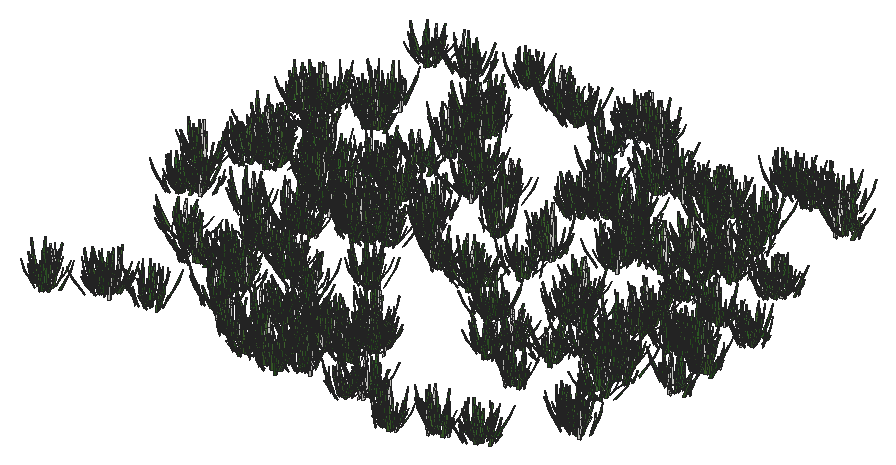
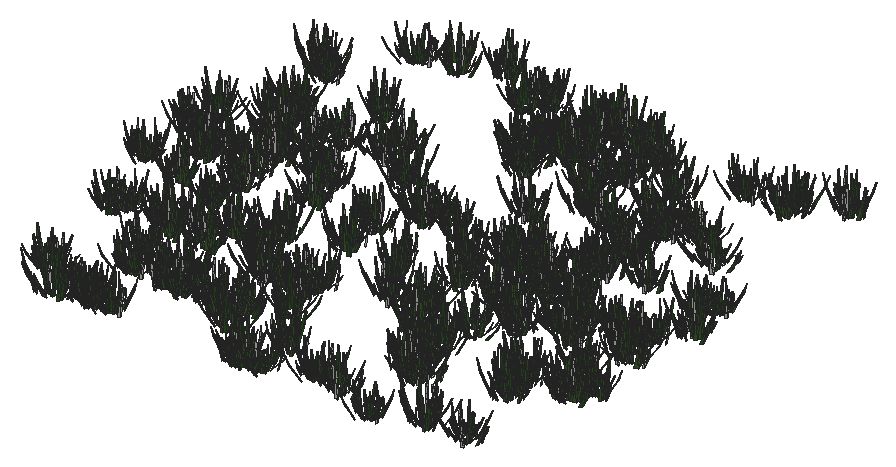
# SketchUp Ruby script. Lengths in inches.
U = 1.inch
M = Sketchup.active_model
def pt(a) = Geom::Point3d.new(a.map { |v| v * U })
def face(e, loops, mat)
  f = e.add_face(loops[0].map { |a| pt(a) })
  loops[1..].each { |l| e.add_face(l.map { |a| pt(a) }).erase! }
  f.material = f.back_material = mat if mat
  f
end
# faces: each face lists its corners as indices into pts; further lists are holes
def faces(e, pts, list, mat = nil) = list.each { |f| face(e, (f[0].is_a?(Array) ? f : [f]).map { |l| l.map { |i| pts[i] } }, mat) }
# xy, xz, yz: faces in a plane at the given z, y or x. An outline is a flat list of corners, or four numbers for a rectangle; further outlines are holes
def ring(l) = l.size == 4 ? [[l[0], l[1]], [l[2], l[1]], [l[2], l[3]], [l[0], l[3]]] : l.each_slice(2).to_a
def flat(e, list, mat, &to3) = list.each { |f| face(e, (f[0].is_a?(Array) ? f : [f]).map { |l| ring(l).map { |u, v| to3.(u, v) } }, mat) }
def xy(e, z, list, mat = nil) = flat(e, list, mat) { |x, y| [x, y, z] }
def xz(e, y, list, mat = nil) = flat(e, list, mat) { |x, z| [x, y, z] }
def yz(e, x, list, mat = nil) = flat(e, list, mat) { |y, z| [x, y, z] }
def lines(e, pts, list) = list.each { |a, b| e.add_line(pt(pts[a]), pt(pts[b])) }
# prism: a flat outline (further loops are holes) pulled along v
def prism(e, loops, v, mat = nil)
  f = face(e, loops, mat); d = Geom::Vector3d.new(v.map { |x| x * U })
  f.pushpull(f.normal.samedirection?(d) ? d.length : -d.length)
end
def box(e, o, s, mat = nil) = prism(e, [[o, [o[0] + s[0], o[1], o[2]], [o[0] + s[0], o[1] + s[1], o[2]], [o[0], o[1] + s[1], o[2]]]], [0, 0, s[2]], mat)
def at(x, y, z, deg = 0) = Geom::Transformation.translation(pt([x, y, z])) * Geom::Transformation.rotation(ORIGIN, Z_AXIS, deg.degrees)
def axes(o, x, y, z) = Geom::Transformation.new([*x, 0, *y, 0, *z, 0, *pt(o).to_a, 1])
def part(name) = M.definitions.add(name)
# library, detail: a bought-in or finely detailed component or shape, given as its bounding box
def library(name, o, s) = part(name).tap { |d| box(d.entities, o, s) }
def detail(e, o, s) = box(e.add_group.entities, o, s)
def put(e, d, t, mat = nil) = e.add_instance(d, t).tap { |i| i.material = mat if mat }
def group(e, t, mat = nil) = e.add_group.tap { |g| g.transformation = t; g.material = mat if mat }.entities
root = M.entities
M.materials.add("Material1").color = [58, 110, 58]
M.materials.add("Material10").color = [48, 100, 38]
M.materials.add("Material3").color = [68, 110, 58]
M.materials.add("Material4").color = [48, 90, 38]
M.materials.add("Material5").color = [68, 110, 48]
M.materials.add("Material6").color = [48, 90, 48]
M.materials.add("Material8").color = [58, 90, 38]
M.materials.add("Material9").color = [68, 100, 58]
c1 = part("grass00")
p = [[-0.6875,0.15,0],[-0.56,0.08,5.52],[-0.04,0.03,2.76],[0.48,-0.02,0],[0.35,-0.02,5.52],[-0.1,-0.14,5.52],
  [-0.12,0.65,8.37],[-0.42,0.65,8.37]]
faces(c1.entities,p,[[0,1,2,3],[3,2,4],[1,5,2],[5,4,2],[1,6,5],[4,5,6],[7,6,1]])
c2 = part("Group16\#1")
put(c2.entities,c1,axes([1.44,-0.61,-0.01],[0.05352,0.12609,0],[-0.10704,0.04543,0.07239],[0.06664,-0.02828,0.11628]),"Material6")
put(c2.entities,c1,axes([0.76,-0.15,-0.01],[0.04676,0.24062,0],[-0.23162,0.04501,0.06642],[0.0652,-0.01267,0.23595]),"Material3")
put(c2.entities,c1,axes([0.79,0.01,-0.01],[-0.00606,0.34651,0],[-0.34381,-0.00602,0.0432],[0.04319,0.00076,0.34386]))
put(c2.entities,c1,axes([1,0.23,-0.01],[-0.07192,0.31144,0],[-0.28722,-0.06632,0.1236],[0.12043,0.02781,0.29478]),"Material5")
put(c2.entities,c1,axes([1.66,0.77,-0.01],[-0.13828,0.29651,0],[-0.21551,-0.1005,0.22471],[0.20365,0.09498,0.23779]),"Material10")
put(c2.entities,c1,axes([0.6875,0.52,-0.01],[-0.18126,0.24051,0],[-0.22746,-0.17142,0.09788],[0.07817,0.05891,0.28481]),"Material5")
put(c2.entities,c1,axes([0.68,0.78,-0.01],[-0.215,0.18688,0],[-0.12385,-0.14248,0.21334],[0.13995,0.16101,0.18878]),"Material3")
put(c2.entities,c1,axes([0.56,1,-0.01],[-0.13756,0.07624,0],[-0.06159,-0.11112,0.0927],[0.04494,0.08108,0.12705]),"Material5")
put(c2.entities,c1,axes([0.2,0.64,-0.01],[-0.23729,0.07254,0],[-0.05711,-0.18681,0.153],[0.04473,0.14632,0.19535]),"Material10")
put(c2.entities,c1,axes([0.0625,0.72,-0.01],[-0.28874,0.02525,0],[-0.02179,-0.24916,0.14647],[0.01276,0.14591,0.25012]),"Material3")
put(c2.entities,c1,axes([-0.08,0.62,-0.01],[-0.34089,-0.04187,0],[0.03255,-0.26504,0.216],[-0.02633,0.21439,0.26703]),"Material10")
put(c2.entities,c1,axes([-0.34,0.98,-0.01],[-0.14314,-0.0493,0],[0.04397,-0.12769,0.06843],[-0.02228,0.0647,0.13505]),"Material10")
put(c2.entities,c1,axes([-0.87,1.45,-0.01],[-0.23488,-0.14114,0],[0.13761,-0.22901,0.06087],[-0.03135,0.05217,0.26717]))
put(c2.entities,c1,axes([-0.72,0.77,-0.01],[-0.14208,-0.13251,0],[0.07209,-0.0773,0.16301],[-0.11118,0.11922,0.1057]),"Material10")
put(c2.entities,c1,axes([-0.62,0.43,-0.01],[-0.14845,-0.21203,0],[0.18654,-0.13061,0.12304],[-0.10079,0.07057,0.22772]),"Material3")
put(c2.entities,c1,axes([-0.68,0.29,-0.01],[-0.13639,-0.32136,0],[0.31723,-0.13464,0.05579],[-0.05136,0.0218,0.34462]),"Material4")
put(c2.entities,c1,axes([-0.64,0.125,-0.01],[-0.0458,-0.23569,0],[0.22124,-0.043,0.08276],[-0.08124,0.01579,0.22538]),"Material1")
put(c2.entities,c1,axes([-1.6,-0.03,-0.01],[0.00576,-0.32897,0],[0.27526,0.00482,0.18018],[-0.18015,-0.00315,0.2753]),"Material5")
put(c2.entities,c1,axes([-1.36,-0.31,-0.01],[0.05718,-0.24765,0],[0.18172,0.04196,0.17267],[-0.16825,-0.03885,0.1865]),"Material10")
put(c2.entities,c1,axes([-1.54,-0.72,-0.01],[0.06537,-0.14017,0],[0.13555,0.06321,0.03939],[-0.0357,-0.01665,0.14956]))
put(c2.entities,c1,axes([-1.19,-0.9,-0.01],[0.09597,-0.12735,0],[0.11214,0.08451,0.07557],[-0.06035,-0.04548,0.14042]),"Material9")
put(c2.entities,c1,axes([-0.47,-0.54,-0.01],[0.11588,-0.10072,0],[0.0618,0.0711,0.12124],[-0.07953,-0.0915,0.0942]))
put(c2.entities,c1,axes([-0.47,-0.84,-0.01],[0.11927,-0.0661,0],[0.06603,0.11913,0.00646],[-0.00313,-0.00565,0.13621]),"Material5")
put(c2.entities,c1,axes([-0.38,-1.24,-0.01],[0.28037,-0.08571,0],[0.0618,0.20215,0.20315],[-0.05939,-0.19428,0.21139]),"Material9")
put(c2.entities,c1,axes([-0.06,-0.66,-0.01],[0.22719,-0.01987,0],[0.01247,0.14255,0.17758],[-0.01547,-0.17691,0.1431]),"Material8")
put(c2.entities,c1,axes([0.11,-0.89,-0.01],[0.14882,0.01828,0],[-0.01058,0.08611,0.12229],[0.01491,-0.12138,0.08676]),"Material6")
put(c2.entities,c1,axes([0.25,-0.72,-0.01],[0.20481,0.07053,0],[-0.06206,0.18022,0.10291],[0.03351,-0.0973,0.1906]),"Material6")
put(c2.entities,c1,axes([0.85,-1.42,-0.01],[0.16481,0.09904,0],[-0.09472,0.15762,0.05616],[0.02893,-0.04814,0.18389]),"Material5")
put(c2.entities,c1,axes([1.01,-1.09,-0.01],[0.21858,0.20385,0],[-0.17495,0.1876,0.15339],[0.10462,-0.11218,0.25652]),"Material10")
put(c2.entities,c1,axes([1.01,-0.71,-0.01],[0.08733,0.12473,0],[-0.06445,0.04512,0.13037],[0.1068,-0.07477,0.07867]),"Material6")
c3 = part("Group15\#1")
put(c3.entities,c2,at(0,0,0))
c4 = part("3darcstudiotree_grass00\#1")
put(c4.entities,c3,at(0,0,0))
put(root,c4,axes([282.91,152.13,0.25],[0.50441,0.65823,0],[-1.00099,0.52844,-0.00074],[-0.00102,0.00054,1.93092]))
put(root,c4,axes([289.35,143.61,0.25],[-0.72293,0.89093,0],[-0.97329,-0.54407,-0.0002],[-0.00027,-0.00015,1.96126]))
put(root,c4,axes([270.9375,158.43,0.25],[0.98465,-0.12149,0],[0.17275,0.96453,-0.00967],[0.00171,0.00957,1.41667]))
put(root,c4,axes([310.59,141.94,0.25],[-0.66862,-0.69978,0],[0.89555,-0.58948,-0.01126],[0.01023,-0.00673,1.32461]))
put(root,c4,axes([321.16,143.97,0.25],[-0.64412,0.82006,0],[-0.86954,-0.47051,-0.00573],[-0.00758,-0.0041,1.63969]))
put(root,c4,axes([331.48,126.1875,0.25],[1.05486,0.41518,0],[-0.38969,0.68208,-0.0026],[-0.00222,0.00389,1.81639]))
put(root,c4,axes([308.12,144.92,0.25],[1.05826,0.20589,0],[-0.22246,0.78769,-0.007],[-0.00256,0.00908,1.56436]))
put(root,c4,axes([275.06,101.88,0.25],[0.19274,0.85396,0],[-1.19074,0.18514,-0.00799],[-0.00978,0.00152,1.50733]))
put(root,c4,axes([269.4,123.27,0.25],[-1.12748,0.03644,0],[-0.03558,-0.7583,-0.00954],[-0.00057,-0.01224,1.41434]))
put(root,c4,axes([280.94,137.52,0.25],[-0.12026,-0.90289,0],[0.9301,-0.08535,-0.00454],[0.00819,-0.00075,1.6986]))
put(root,c4,axes([307.15,99.47,0.25],[-0.42808,-0.69918,0],[0.99835,-0.42109,-0.00876],[0.01015,-0.00428,1.45672]))
put(root,c4,axes([291.02,126.91,0.25],[0.95151,-0.32357,0],[0.35722,0.72367,-0.00746],[0.00458,0.00929,1.52751]))
put(root,c4,axes([293.13,130.49,0.25],[-0.53335,-0.60654,0],[0.85943,-0.52062,-0.00015],[0.00022,-0.00014,1.94435]))
put(root,c4,axes([270.78,140.02,0.25],[-1.00771,-0.1754,0],[0.24056,-0.95209,-0.00999],[0.00242,-0.00957,1.38276]))
put(root,c4,axes([287.26,115.55,0.25],[0.92934,-0.33875,0],[0.46115,0.87155,-0.00525],[0.00304,0.00574,1.64886]))
put(root,c4,axes([273.91,114.75,0.25],[1.28779,-0.10782,0],[0.12101,0.99564,-0.01121],[0.00122,0.01004,1.30781]))
put(root,c4,axes([312.21,152.58,0.25],[0.38901,0.72653,0],[-1.07347,0.39596,-0.00487],[-0.00632,0.00233,1.66894]))
put(root,c4,axes([290.12,102.31,0.25],[-0.67966,0.71325,0],[-0.73342,-0.48146,-0.01059],[-0.0119,-0.00781,1.33934]))
put(root,c4,axes([298.05,99.55,0.25],[0.27356,-0.98457,0],[1.03655,0.1984,-0.00305],[0.00494,0.00095,1.76865]))
put(root,c4,axes([284.49,147.29,0.25],[-0.09469,-0.83837,0],[1.12214,-0.08731,-0.00863],[0.01106,-0.00086,1.44957]))
put(root,c4,axes([281.7,160.85,0.25],[0.75518,0.45958,0],[-0.62327,0.70554,-0.01003],[-0.0077,0.00872,1.36834]))
put(root,c4,axes([328.78,143.63,0.25],[-0.91105,0.16514,0],[-0.20716,-0.78732,-0.01018],[-0.00304,-0.01156,1.35975]))
put(root,c4,axes([325.4,119.33,0.25],[1.09165,0.06839,0],[-0.09508,1.04561,-0.00004],[0,0.00005,1.93334]))
put(root,c4,axes([298.02,135.62,0.25],[-0.36557,1.02345,0],[-0.8678,-0.21354,-0.00114],[-0.00227,-0.00056,1.86907]))
put(root,c4,axes([305.18,134.9,0.25],[-0.30893,0.95853,0],[-1.11215,-0.24693,-0.00132],[-0.00206,-0.00046,1.858]))
put(root,c4,axes([292.13,107.28,0.25],[0.76845,0.56751,0],[-0.64535,0.60199,-0.00943],[-0.00899,0.00839,1.39243]))
put(root,c4,axes([271.72,132.0625,0.25],[1.0465,-0.407,0],[0.49619,0.87892,-0.00986],[0.00489,0.00867,1.36783]))
put(root,c4,axes([283.01,118.25,0.25],[-0.20632,-0.8847,0],[0.88885,-0.1428,-0.00678],[0.01135,-0.00182,1.54322]))
put(root,c4,axes([325.72,157.09,0.25],[-1.09338,0.54066,0],[-0.57925,-0.80699,-0.00882],[-0.00569,-0.00792,1.42641]))
put(root,c4,axes([299.33,106.58,0.25],[0.13337,-0.79747,0],[0.99583,0.11473,-0.0013],[0.00238,0.00027,1.85519]))
put(root,c4,axes([294.85,118.7,0.25],[0.94591,-0.15419,0],[0.20231,0.855,-0.00241],[0.00079,0.00334,1.79003]))
put(root,c4,axes([309.11,101.2,0.25],[-0.922,0.2214,0],[-0.33581,-0.96337,-0.00573],[-0.00211,-0.00605,1.59925]))
put(root,c4,axes([300.93,111.99,0.25],[-0.02731,0.7764,0],[-1.11819,-0.0271,-0.00454],[-0.00675,-0.00016,1.66362]))
put(root,c4,axes([301.63,109.125,0.25],[1.17253,-0.36863,0],[0.38926,0.85297,-0.01068],[0.00451,0.00989,1.31138]))
put(root,c4,axes([284.84,144.8125,0.25],[-1.03711,0.60741,0],[-0.57029,-0.67081,0],[0,0,1.91868]))
put(root,c4,axes([269.53,135.08,0.25],[0.08651,0.8649,0],[-0.95463,0.06578,-0.00998],[-0.01401,0.00097,1.34846]))
put(root,c4,axes([322.04,124.97,0.25],[1.09717,-0.44005,0],[0.48495,0.83295,-0.00312],[0.00212,0.00364,1.73901]))
put(root,c4,axes([321.32,120.85,0.25],[-1.24748,0.17318,0],[-0.19972,-0.9911,-0.00717],[-0.00147,-0.00731,1.50735]))
put(root,c4,axes([290.66,157.8125,0.25],[0.8671,0.70801,0],[-0.65077,0.54905,-0.00671],[-0.00777,0.00656,1.53359]))
put(root,c4,axes([314.68,97.2,0.25],[-0.51158,0.6582,0],[-0.86214,-0.46162,-0.00439],[-0.00599,-0.00321,1.66469]))
put(root,c4,axes([313.23,115.06,0.25],[1.08099,-0.39691,0],[0.39768,0.74614,-0.00969],[0.00543,0.01018,1.36001]))
put(root,c4,axes([270.8125,133.48,0.25],[0.81346,-0.68452,0],[0.72164,0.59078,-0.00165],[0.0021,0.00172,1.81884]))
put(root,c4,axes([298.44,107.12,0.25],[-1.17544,-0.44269,0],[0.50763,-0.92855,-0.00153],[0.00094,-0.00171,1.82565]))
put(root,c4,axes([304.65,154.95,0.25],[-1.24894,0.29251,0],[-0.33363,-0.98132,-0.00145],[-0.00059,-0.00173,1.8291]))
put(root,c4,axes([317.84,160.07,0.25],[-0.52705,-0.66139,0],[0.86003,-0.47213,-0.00554],[0.00715,-0.00392,1.59445]))
put(root,c4,axes([316.41,125.69,0.25],[1.23649,-0.09818,0],[0.09258,0.80317,-0.00501],[0.0008,0.00691,1.62495]))
put(root,c4,axes([269.68,97.99,0.25],[0.86217,-0.23787,0],[0.33362,0.83302,-0.00205],[0.0011,0.00274,1.79239]))
put(root,c4,axes([321.27,131.9,0.25],[-0.25458,-1.00074,0],[1.03583,-0.18153,-0.00703],[0.0098,-0.00172,1.50812]))
put(root,c4,axes([278.7,130.49,0.25],[0.20448,0.82006,0],[-1.18765,0.20401,-0.00233],[-0.00333,0.00057,1.77271]))
put(root,c4,axes([281.55,128.04,0.25],[-1.07124,-0.38073,0],[0.48875,-0.94735,-0.00601],[0.00298,-0.00577,1.5624]))
put(root,c4,axes([282.87,130.62,0.25],[-0.05369,0.96357,0],[-1.07942,-0.04143,-0.00948],[-0.01196,-0.00046,1.36423]))
put(root,c4,axes([296.21,159.79,0.25],[0.1849,0.98535,0],[-0.91329,0.11806,-0.00889],[-0.01328,0.00172,1.39664]))
put(root,c4,axes([284.21,140.66,0.25],[-0.99074,0.57217,0],[-0.59485,-0.70958,-0.01001],[-0.0073,-0.00871,1.32974]))
put(root,c4,axes([319.63,159.54,0.25],[0.8015,-0.60544,0],[0.70687,0.64466,-0.00947],[0.00825,0.00753,1.36019]))
put(root,c4,axes([323.63,100.51,0.25],[0.93467,0.70089,0],[-0.63056,0.57928,-0.00582],[-0.00649,0.00596,1.56404]))
put(root,c4,axes([291.74,104.86,0.25],[1.02854,0.04253,0],[-0.06022,1.00326,-0.00527],[-0.00035,0.00575,1.59512]))
put(root,c4,axes([325.32,122.25,0.25],[-0.6501,0.74781,0],[-0.74806,-0.448,-0.00844],[-0.01048,-0.00628,1.41311]))
put(root,c4,axes([304.45,144.76,0.25],[0.35275,1.00784,0],[-0.87459,0.21088,-0.00931],[-0.01338,0.00323,1.3628]))
put(root,c4,axes([328.49,128.57,0.25],[0.26515,-0.78836,0],[1.06508,0.24678,-0.00232],[0.00355,0.00082,1.76107]))
put(root,c4,axes([302.71,105.32,0.25],[0.01219,-0.80747,0],[0.97741,0.01016,-0.00992],[0.01341,0.00014,1.32167]))
put(root,c4,axes([282.6,136.18,0.25],[0.02256,-0.76708,0],[0.99939,0.02025,-0.00377],[0.00628,0.00013,1.66719]))
put(root,c4,axes([273.51,145.6,0.25],[0.03239,0.79334,0],[-0.95916,0.02698,-0.00216],[-0.00395,0.00011,1.758]))
put(root,c4,axes([314.2,149.74,0.25],[1.1608,-0.08489,0],[0.10873,1.02421,-0.00682],[0.00072,0.00679,1.49182]))
put(root,c4,axes([278.02,111.74,0.25],[0.64824,-0.72307,0],[1.01392,0.6262,-0.00846],[0.00749,0.00463,1.39582]))
put(root,c4,axes([302.77,144.9375,0.25],[0.33936,-0.6925,0],[0.93639,0.31613,-0.0011],[0.00183,0.00062,1.80895]))
put(root,c4,axes([299.12,104.58,0.25],[0.29729,0.96356,0],[-1.16739,0.24812,-0.00469],[-0.00605,0.00129,1.60422]))
put(root,c4,axes([308.64,152.59,0.25],[-1.11491,0.05093,0],[-0.05949,-0.897,-0.00024],[-0.00002,-0.00035,1.85086]))
put(root,c4,axes([282.42,151.08,0.25],[1.12331,-0.17686,0],[0.22956,1.00446,-0.00778],[0.00167,0.00732,1.42033]))
put(root,c4,axes([298.51,159.97,0.25],[-0.82115,0.82106,0],[-0.84331,-0.58102,-0.00469],[-0.00525,-0.00362,1.59556]))
put(root,c4,axes([281.8,113.59,0.25],[0.60833,0.71141,0],[-0.90067,0.53057,-0.0048],[-0.00563,0.00331,1.58899]))
put(root,c4,axes([290.63,114.14,0.25],[-1.13273,-0.38933,0],[0.36267,-0.72691,-0.00358],[0.00239,-0.00479,1.65637]))
put(root,c4,axes([307.26,144.93,0.25],[0.85693,-0.40974,0],[0.58297,0.83992,-0.00508],[0.00341,0.00491,1.56982]))
put(root,c4,axes([275.03,144.54,0.25],[0.68162,-0.66038,0],[0.80266,0.57074,-0.00664],[0.00706,0.00502,1.48048]))
put(root,c4,axes([294.92,140.84,0.25],[1.05914,-0.19721,0],[0.20058,0.74214,-0.00297],[0.0012,0.00442,1.68702]))
put(root,c4,axes([330.43,107.9375,0.25],[-0.98651,-0.16387,0],[0.19035,-0.78945,-0.00178],[0.00063,-0.00262,1.75352]))
put(root,c4,axes([328.3,129.37,0.25],[-1.05274,-0.12925,0],[0.13693,-0.76834,-0.00812],[0.00176,-0.0099,1.3892]))
put(root,c4,axes([284.96,110.65,0.25],[0.88711,-0.56782,0],[0.63485,0.68327,-0.00737],[0.00619,0.00667,1.42978]))
put(root,c4,axes([276.31,158.48,0.25],[-1.14331,0.05364,0],[-0.05986,-0.87896,-0.00256],[-0.00023,-0.00341,1.70382]))
put(root,c4,axes([299.64,159.87,0.25],[-0.54292,0.78663,0],[-0.90263,-0.42918,-0.00674],[-0.00823,-0.00391,1.46389]))
put(root,c4,axes([276.29,122.46,0.25],[0.94405,-0.15498,0],[0.18211,0.7642,-0.00259],[0.00091,0.00381,1.70099]))
put(root,c4,axes([315.91,139.95,0.25],[-0.48741,0.93296,0],[-1.05725,-0.38051,-0.00354],[-0.00464,-0.00167,1.64409]))
put(root,c4,axes([275.4,136,0.25],[0.21629,0.84043,0],[-1.16779,0.20705,-0.00171],[-0.00245,0.00043,1.74655]))
put(root,c4,axes([322.29,128.64,0.25],[-0.36784,-0.88953,0],[1.15738,-0.3297,-0.00214],[0.00284,-0.00081,1.72072]))
put(root,c4,axes([293.51,110.4375,0.25],[-1.17507,0.21035,0],[-0.23348,-0.89852,-0.00845],[-0.00219,-0.00841,1.35873]))
put(root,c4,axes([302.2,143.18,0.25],[0.22975,0.9189,0],[-1.03043,0.17748,-0.00381],[-0.00574,0.00099,1.62105]))
put(root,c4,axes([308.7,121.16,0.25],[-0.85469,-0.67309,0],[0.77805,-0.68062,-0.00166],[0.00176,-0.00154,1.74215]))
put(root,c4,axes([268.81,145.05,0.25],[-0.27616,-0.86577,0],[1.02945,-0.22622,-0.00114],[0.00183,-0.0004,1.77079]))
put(root,c4,axes([305.19,151.87,0.25],[-0.61947,0.56293,0],[-0.94889,-0.71934,-0.00484],[-0.00433,-0.00329,1.55938]))
put(root,c4,axes([322.53,160.74,0.25],[-1.24447,-0.28446,0],[0.31956,-0.9631,-0.00177],[0.00068,-0.00204,1.73275]))
put(root,c4,axes([293.75,100.29,0.25],[-0.22832,-0.85091,0],[0.88743,-0.16404,-0.00779],[0.01162,-0.00215,1.38852]))
put(root,c4,axes([273.38,148.79,0.25],[-0.83499,-0.64599,0],[0.79643,-0.70919,-0.00052],[0.00054,-0.00048,1.79691]))
put(root,c4,axes([322.45,142.68,0.25],[-0.04735,-0.76009,0],[1.23763,-0.05311,-0.00424],[0.00542,-0.00023,1.58408]))
put(root,c4,axes([275.55,133.11,0.25],[0.91279,0.18953,0],[-0.30366,1.00751,-0.00744],[-0.00202,0.00671,1.4009]))
put(root,c4,axes([318.88,152.41,0.25],[1.01528,0.45064,0],[-0.45874,0.712,-0.00407],[-0.00314,0.00487,1.59208]))
put(root,c4,axes([303.01,109.39,0.25],[-1.13287,-0.12959,0],[0.15909,-0.95815,-0.00876],[0.00136,-0.00817,1.32289]))
put(root,c4,axes([285.87,131.26,0.25],[-0.88736,-0.41088,0],[0.44535,-0.66258,-0.00653],[0.00504,-0.0075,1.4475]))
put(root,c4,axes([269.17,131.0625,0.25],[0.25514,0.96804,0],[-0.9952,0.1807,-0.00261],[-0.00418,0.00076,1.6704]))
put(root,c4,axes([289.1,126.18,0.25],[-0.44633,-0.99757,0],[1.12785,-0.34763,-0.00006],[0.00009,-0.00003,1.81412]))
put(root,c4,axes([319.03,111.95,0.25],[-0.82209,0.57363,0],[-0.58018,-0.5728,-0.00081],[-0.00102,-0.00101,1.76997]))
put(root,c4,axes([311.71,137.02,0.25],[-0.88615,-0.35401,0],[0.55711,-0.96071,-0.00367],[0.00199,-0.00343,1.60507]))
put(root,c4,axes([281.38,111.64,0.25],[-0.91472,0.10782,0],[-0.15447,-0.90277,-0.00819],[-0.00141,-0.00824,1.3463]))
put(root,c4,axes([268.28,135.17,0.25],[0.94171,-0.68989,0],[0.84127,0.7911,-0.00351],[0.00294,0.00276,1.60808]))
put(root,c4,axes([313.61,129.92,0.25],[-0.40567,0.73084,0],[-1.08875,-0.41633,-0.00587],[-0.00655,-0.00251,1.47291]))
put(root,c4,axes([291.48,133.51,0.25],[0.13967,0.98095,0],[-1.09726,0.10763,-0.00527],[-0.00712,0.0007,1.50433]))
put(root,c4,axes([319.82,141.14,0.25],[1.1188,-0.42752,0],[0.39769,0.71696,-0.00355],[0.0025,0.0045,1.60125]))
put(root,c4,axes([278.1875,134.84,0.25],[1.09585,0.42025,0],[-0.42166,0.75746,-0.00765],[-0.00435,0.00782,1.36419]))
put(root,c4,axes([318.79,118.19,0.25],[0.1848,-1.04083,0],[1.14507,0.14006,-0.00777],[0.00898,0.0011,1.3523]))
put(root,c4,axes([328.46,109.12,0.25],[0.59987,0.61343,0],[-0.75132,0.50614,-0.00448],[-0.00553,0.00373,1.5389]))
put(root,c4,axes([281.3,123.12,0.25],[1.15328,0.17206,0],[-0.20698,0.95574,-0.00017],[-0.00005,0.00022,1.78268]))
put(root,c4,axes([332.61,121.17,0.25],[-1.09262,0.49269,0],[-0.46211,-0.70599,-0.00649],[-0.00455,-0.00695,1.42064]))
put(root,c4,axes([280.91,118.46,0.25],[-0.07181,1.06171,0],[-0.90531,-0.04218,-0.00552],[-0.00896,-0.00042,1.47331]))
put(root,c4,axes([296.46,100.34,0.25],[-0.45538,0.84316,0],[-1.13015,-0.4205,-0.00369],[-0.00429,-0.0016,1.57624]))
put(root,c4,axes([321.32,136.26,0.25],[-0.59214,-0.62104,0],[0.85394,-0.5609,-0.00813],[0.00774,-0.00508,1.32168]))
put(root,c4,axes([266.68,142.72,0.25],[0.7933,-0.65681,0],[0.66603,0.55418,-0.0036],[0.00426,0.00354,1.5794]))
put(root,c4,axes([268.08,144.77,0.25],[-0.60977,0.92433,0],[-1.13036,-0.51371,-0.00813],[-0.0073,-0.00332,1.31962]))
put(root,c4,axes([285.63,105.95,0.25],[1.05714,0.31332,0],[-0.39246,0.91221,-0.00059],[-0.0003,0.00069,1.74794]))
put(root,c4,axes([283.35,123.28,0.25],[-0.61937,0.6357,0],[-0.73523,-0.49349,-0.00747],[-0.00832,-0.00558,1.35493]))
put(root,c4,axes([297.02,104.625,0.25],[0.23174,-0.99836,0],[1.09052,0.17439,-0.00212],[0.00311,0.0005,1.6588]))
put(root,c4,axes([326.68,127.36,0.25],[1.10112,-0.18566,0],[0.18814,0.76869,-0.00331],[0.00111,0.00453,1.58887]))
put(root,c4,axes([267.8125,122.04,0.25],[0.87367,0.58915,0],[-0.62574,0.63925,-0.0068],[-0.00599,0.00612,1.38619]))
put(root,c4,axes([327.13,134.73,0.25],[-0.507,0.62163,0],[-0.90165,-0.50661,-0.00267],[-0.00329,-0.00185,1.62102]))
put(root,c4,axes([266.54,127.16,0.25],[-0.59205,0.84341,0],[-1.07578,-0.52024,-0.00219],[-0.0025,-0.00121,1.64693]))
put(root,c4,axes([298.16,126.125,0.25],[-1.03316,0.63037,0],[-0.56211,-0.63467,-0.00523],[-0.00481,-0.00543,1.47184]))
put(root,c4,axes([284.83,150.94,0.25],[0.14422,-0.8922,0],[0.92409,0.1029,-0.00096],[0.00175,0.0002,1.71349]))
put(root,c4,axes([302.83,125,0.25],[1.26299,-0.07031,0],[0.08353,1.03367,-0.00473],[0.00038,0.0047,1.49489]))
put(root,c4,axes([315.84,160.02,0.25],[0.79545,0.558,0],[-0.68587,0.67356,-0.00305],[-0.00294,0.00289,1.58836]))
put(root,c4,axes([327.2,115.4375,0.25],[1.01984,-0.35977,0],[0.47461,0.92683,-0.00549],[0.00255,0.00498,1.44062]))
put(root,c4,axes([291.42,139.35,0.25],[-1.18295,-0.10695,0],[0.11742,-0.89467,-0.0047],[0.0007,-0.00531,1.4854]))
put(root,c4,axes([285.49,127.48,0.25],[0.08851,-0.92908,0],[1.01371,0.06653,-0.00365],[0.00552,0.00036,1.54435]))
put(root,c4,axes([316.63,143.52,0.25],[-0.52392,0.89266,0],[-1.16536,-0.47119,-0.00711],[-0.00663,-0.00268,1.34501]))
put(root,c4,axes([296.59,155.25,0.25],[-0.43456,-0.69113,0],[0.9828,-0.42571,-0.00435],[0.00522,-0.00226,1.50222]))
put(root,c4,axes([332.59,125.9,0.25],[0.4273,-0.70081,0],[0.96229,0.4042,-0.00728],[0.00802,0.00337,1.33141]))
put(root,c4,axes([312.16,138.84,0.25],[0.87013,0.6898,0],[-0.67419,0.58586,-0.00574],[-0.00576,0.005,1.41814]))
put(root,c4,axes([287.21,158.7,0.25],[1.25697,-0.25945,0],[0.23262,0.77638,-0.00031],[0.00013,0.00045,1.72722]))
put(root,c4,axes([319.2,99.41,0.25],[-0.84075,0.53756,0],[-0.61206,-0.65947,-0.00087],[-0.00089,-0.00096,1.68429]))
put(root,c4,axes([286,134.71,0.25],[0.14412,-0.96609,0],[1.17635,0.1209,-0.00236],[0.00316,0.00033,1.5989]))
put(root,c4,axes([327.83,142.49,0.25],[0.40689,0.7371,0],[-1.08542,0.41277,-0.00338],[-0.00397,0.00151,1.53978]))
put(root,c4,axes([280.17,101.72,0.25],[0.90041,0.40433,0],[-0.57696,0.88512,-0.00222],[-0.0014,0.00215,1.6055]))
put(root,c4,axes([301.24,148.9375,0.25],[-1.02824,0.40165,0],[-0.4708,-0.83029,-0.0027],[-0.00164,-0.00289,1.57765]))
put(root,c4,axes([314.25,152.5625,0.25],[0.68619,-0.5241,0],[0.81095,0.73144,-0.00074],[0.00071,0.00064,1.68668]))
put(root,c4,axes([313.63,118.1875,0.25],[1.26513,-0.00839,0],[0.00953,0.99103,-0.00522],[0.00005,0.00519,1.42947]))
put(root,c4,axes([314.48,125.64,0.25],[0.22292,-0.77284,0],[0.99816,0.19834,-0.00366],[0.00525,0.00104,1.51551]))
put(root,c4,axes([326.54,119.47,0.25],[1.18464,0.32101,0],[-0.37446,0.95197,-0.00124],[-0.00053,0.00134,1.65228]))
put(root,c4,axes([305.62,130.04,0.25],[-0.13854,-0.80282,0],[1.25541,-0.14924,-0.00214],[0.00267,-0.00032,1.59988]))
put(root,c4,axes([320.9375,148.32,0.25],[0.47076,0.7228,0],[-0.97919,0.43934,-0.00296],[-0.00363,0.00163,1.55057]))
put(root,c4,axes([287.34,125.62,0.25],[0.21502,-0.84506,0],[1.00632,0.1764,-0.00249],[0.00372,0.00065,1.57305]))
put(root,c4,axes([288.59,128.71,0.25],[-1.08251,0.40727,0],[-0.4654,-0.85219,-0.00714],[-0.00341,-0.00624,1.30481]))
put(root,c4,axes([300.53,100.8,0.25],[-0.76588,-0.47402,0],[0.65706,-0.73136,-0.00029],[0.00027,-0.0003,1.69542]))
put(root,c4,axes([302.6,126.06,0.25],[-1.20669,0.211,0],[-0.22141,-0.87229,-0.00142],[-0.00044,-0.00175,1.63114]))
put(root,c4,axes([303.6875,108.22,0.25],[-0.62878,-0.64022,0],[0.80993,-0.54799,-0.00371],[0.00412,-0.00279,1.4993]))
put(root,c4,axes([274.74,100.61,0.25],[-0.95729,-0.48064,0],[0.67257,-0.92284,-0.00291],[0.00179,-0.00245,1.54121]))
put(root,c4,axes([332.5625,133.33,0.25],[0.52077,0.69547,0],[-0.8234,0.42476,-0.00184],[-0.00258,0.00133,1.60144]))
